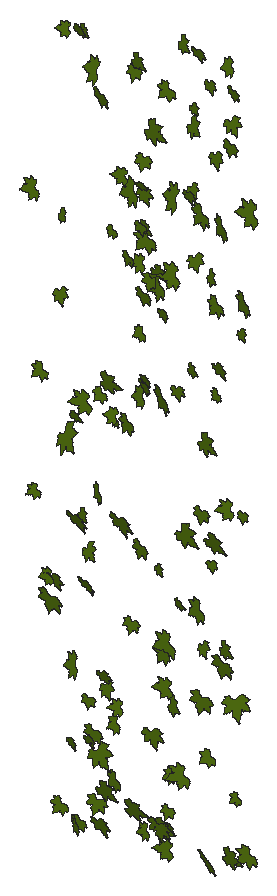
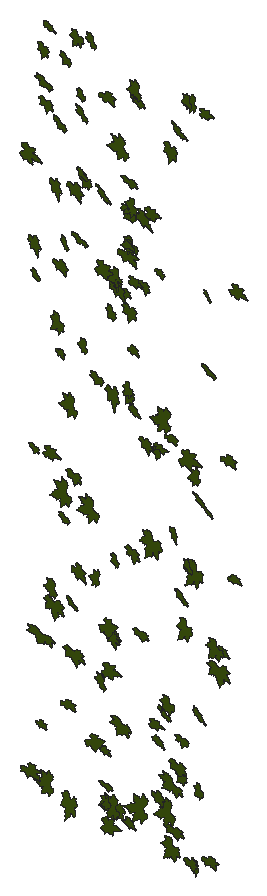
# SketchUp Ruby script. Lengths in inches.
U = 1.inch
M = Sketchup.active_model
def pt(a) = Geom::Point3d.new(a.map { |v| v * U })
def face(e, loops, mat)
  f = e.add_face(loops[0].map { |a| pt(a) })
  loops[1..].each { |l| e.add_face(l.map { |a| pt(a) }).erase! }
  f.material = f.back_material = mat if mat
  f
end
# faces: each face lists its corners as indices into pts; further lists are holes
def faces(e, pts, list, mat = nil) = list.each { |f| face(e, (f[0].is_a?(Array) ? f : [f]).map { |l| l.map { |i| pts[i] } }, mat) }
# xy, xz, yz: faces in a plane at the given z, y or x. An outline is a flat list of corners, or four numbers for a rectangle; further outlines are holes
def ring(l) = l.size == 4 ? [[l[0], l[1]], [l[2], l[1]], [l[2], l[3]], [l[0], l[3]]] : l.each_slice(2).to_a
def flat(e, list, mat, &to3) = list.each { |f| face(e, (f[0].is_a?(Array) ? f : [f]).map { |l| ring(l).map { |u, v| to3.(u, v) } }, mat) }
def xy(e, z, list, mat = nil) = flat(e, list, mat) { |x, y| [x, y, z] }
def xz(e, y, list, mat = nil) = flat(e, list, mat) { |x, z| [x, y, z] }
def yz(e, x, list, mat = nil) = flat(e, list, mat) { |y, z| [x, y, z] }
def lines(e, pts, list) = list.each { |a, b| e.add_line(pt(pts[a]), pt(pts[b])) }
# prism: a flat outline (further loops are holes) pulled along v
def prism(e, loops, v, mat = nil)
  f = face(e, loops, mat); d = Geom::Vector3d.new(v.map { |x| x * U })
  f.pushpull(f.normal.samedirection?(d) ? d.length : -d.length)
end
def box(e, o, s, mat = nil) = prism(e, [[o, [o[0] + s[0], o[1], o[2]], [o[0] + s[0], o[1] + s[1], o[2]], [o[0], o[1] + s[1], o[2]]]], [0, 0, s[2]], mat)
def at(x, y, z, deg = 0) = Geom::Transformation.translation(pt([x, y, z])) * Geom::Transformation.rotation(ORIGIN, Z_AXIS, deg.degrees)
def axes(o, x, y, z) = Geom::Transformation.new([*x, 0, *y, 0, *z, 0, *pt(o).to_a, 1])
def part(name) = M.definitions.add(name)
# library, detail: a bought-in or finely detailed component or shape, given as its bounding box
def library(name, o, s) = part(name).tap { |d| box(d.entities, o, s) }
def detail(e, o, s) = box(e.add_group.entities, o, s)
def put(e, d, t, mat = nil) = e.add_instance(d, t).tap { |i| i.material = mat if mat }
def group(e, t, mat = nil) = e.add_group.tap { |g| g.transformation = t; g.material = mat if mat }.entities
root = M.entities
M.materials.add("[Vegetation Blur 03]").color = [83, 114, 18]
c1 = part("ivy")
xy(c1.entities,0,[[0.782,0,0.786,0,0.787,0.005,0.789,0.009,0.821,0.072,0.875,0.147,1.001,0.272,1.073,0.331,1.137,0.363,1.178,0.379,1.223,0.384,1.272,0.383,1.311,0.374,1.36,0.355,1.399,0.334,1.491,0.285,1.541,0.244,1.583,0.199,1.617,0.15,1.64,0.128,1.662,0.115,1.717,0.105,1.745,0.093,1.784,0.054,1.819,0.057,1.854,0.064,1.882,0.075,1.896,0.074,1.91,0.071,1.937,0.063,1.964,0.053,1.99,0.038,2.016,0.015,2.034,0.002,2.04,0,2.038,0.003,2.036,0.007,2.033,0.038,2.036,0.068,2.045,0.1,2.055,0.116,2.064,0.123,2.077,0.129,2.088,0.129,2.106,0.132,2.118,0.13,2.179,0.132,2.207,0.133,2.225,0.133,2.242,0.138,2.22,0.162,2.207,0.186,2.206,0.213,2.212,0.236,2.228,0.262,2.247,0.274,2.298,0.283,2.355,0.294,2.37,0.296,2.376,0.295,2.377,0.3,2.377,0.303,2.385,0.329,2.411,0.37,2.426,0.392,2.449,0.407,2.511,0.426,2.561,0.444,2.619,0.466,2.589,0.469,2.561,0.476,2.501,0.5,2.449,0.516,2.424,0.523,2.401,0.535,2.377,0.556,2.372,0.568,2.36,0.575,2.268,0.586,2.225,0.592,2.207,0.599,2.194,0.61,2.143,0.65,2.13,0.664,2.122,0.682,2.123,0.7,2.13,0.719,2.148,0.75,2.17,0.781,2.195,0.807,2.221,0.828,2.284,0.874,2.291,0.88,2.288,0.887,2.276,0.9,2.267,0.916,2.265,0.933,2.273,0.967,2.292,1.002,2.313,1.03,2.334,1.054,2.348,1.067,2.358,1.074,2.363,1.076,2.362,1.081,2.35,1.094,2.347,1.11,2.35,1.143,2.359,1.18,2.385,1.254,2.415,1.324,2.448,1.393,2.45,1.4,2.446,1.398,2.44,1.394,2.427,1.383,2.402,1.36,2.376,1.339,2.345,1.324,2.305,1.309,2.282,1.303,2.273,1.306,2.245,1.294,2.212,1.287,2.187,1.291,2.163,1.301,2.142,1.316,2.134,1.327,2.124,1.325,2.09,1.292,2.053,1.259,2.014,1.234,1.973,1.215,1.954,1.21,1.931,1.208,1.909,1.212,1.893,1.22,1.879,1.233,1.872,1.248,1.867,1.281,1.864,1.319,1.821,1.258,1.773,1.197,1.726,1.141,1.698,1.121,1.679,1.116,1.666,1.117,1.647,1.122,1.632,1.129,1.62,1.141,1.617,1.154,1.617,1.219,1.621,1.254,1.623,1.268,1.623,1.281,1.618,1.314,1.606,1.346,1.603,1.375,1.607,1.403,1.603,1.467,1.599,1.499,1.605,1.525,1.614,1.552,1.629,1.577,1.635,1.589,1.629,1.587,1.618,1.582,1.596,1.566,1.581,1.556,1.568,1.552,1.557,1.55,1.545,1.553,1.531,1.562,1.522,1.572,1.504,1.591,1.486,1.611,1.474,1.631,1.457,1.666,1.455,1.684,1.457,1.698,1.452,1.715,1.444,1.728,1.424,1.754,1.419,1.772,1.423,1.786,1.434,1.819,1.444,1.848,1.446,1.855,1.44,1.861,1.43,1.867,1.386,1.904,1.349,1.948,1.326,1.973,1.31,1.995,1.288,2.048,1.284,2.153,1.287,2.254,1.284,2.255,1.282,2.253,1.278,2.247,1.274,2.237,1.266,2.216,1.226,2.125,1.208,2.076,1.184,2.033,1.155,1.984,1.135,1.942,1.111,1.899,1.083,1.861,1.053,1.85,1.059,1.83,1.061,1.809,1.056,1.79,1.049,1.767,1.04,1.749,1.018,1.733,0.994,1.726,0.942,1.734,0.95,1.6875,0.944,1.645,0.932,1.608,0.911,1.585,0.881,1.58,0.854,1.582,0.828,1.588,0.785,1.618,0.773,1.625,0.775,1.614,0.779,1.598,0.796,1.502,0.818,1.402,0.861,1.283,0.882,1.224,0.894,1.174,0.892,1.148,0.886,1.123,0.881,1.107,0.872,1.099,0.849,1.094,0.818,1.092,0.789,1.098,0.762,1.107,0.753,1.113,0.721,1.139,0.698,1.163,0.678,1.194,0.665,1.224,0.628,1.28,0.612,1.312,0.606,1.327,0.606,1.314,0.599,1.282,0.594,1.267,0.581,1.256,0.544,1.245,0.512,1.244,0.473,1.249,0.444,1.256,0.382,1.288,0.339,1.306,0.324,1.316,0.317,1.324,0.309,1.326,0.27,1.314,0.227,1.313,0.185,1.3125,0.152,1.317,0.122,1.328,0.092,1.345,0.073,1.353,0.079,1.338,0.092,1.308,0.117,1.249,0.13,1.215,0.139,1.164,0.147,1.148,0.157,1.136,0.163,1.122,0.174,1.086,0.177,1.067,0.182,1.054,0.186,1.043,0.191,1.038,0.211,1.028,0.237,1.005,0.25,0.974,0.253,0.96,0.25,0.944,0.242,0.914,0.243,0.906,0.249,0.902,0.26,0.894,0.289,0.88,0.307,0.873,0.322,0.862,0.364,0.799,0.403,0.738,0.431,0.709,0.439,0.691,0.441,0.678,0.4375,0.66,0.428,0.645,0.394,0.623,0.303,0.594,0.255,0.581,0.214,0.577,0.179,0.573,0.173,0.568,0.175,0.561,0.167,0.55,0.141,0.523,0.113,0.503,0.077,0.49,0.045,0.486,0.026,0.485,0.019,0.486,0.011,0.483,0,0.471,0.014,0.467,0.044,0.455,0.058,0.447,0.07,0.438,0.097,0.411,0.125,0.394,0.158,0.377,0.174,0.366,0.182,0.359,0.185,0.361,0.242,0.331,0.253,0.316,0.258,0.303,0.262,0.283,0.274,0.278,0.308,0.274,0.341,0.252,0.366,0.226,0.366,0.222,0.37,0.22,0.38,0.221,0.395,0.221,0.425,0.216,0.45,0.207,0.465,0.192,0.473,0.178,0.484,0.15,0.489,0.116,0.483,0.089,0.468,0.058,0.45,0.035,0.435,0.018,0.429,0.011,0.434,0.012,0.438,0.014,0.469,0.019,0.542,0.016,0.581,0.015,0.612,0.027,0.68,0.055,0.696,0.057,0.712,0.052,0.73,0.045,0.741,0.036,0.766,0.014]])
put(root,c1,axes([124.42,173.8,43.62],[0.34903,-0.06561,0.18456],[0.21828,-0.15404,-0.28357],[-0.06714,-0.84183,0.0375]),"[Vegetation Blur 03]")
put(root,c1,axes([125.8,173.8,49.1875],[0.2034,-0.19719,-0.25526],[-0.32297,-0.00076,-0.17132],[-0.05192,-0.76775,0.06573]),"[Vegetation Blur 03]")
put(root,c1,axes([116.46,173.8,6.22],[0.37274,-0.27698,-0.10257],[-0.11734,0.09274,-0.32343],[-0.14192,-0.80413,-0.00197]),"[Vegetation Blur 03]")
put(root,c1,axes([116.69,173.8,14.82],[0.25932,-0.29593,-0.35358],[-0.43934,0.11655,-0.22996],[-0.12392,-1.03246,0.07539]),"[Vegetation Blur 03]")
put(root,c1,axes([124.1,173.8,23.1],[0.31154,-0.18802,0.42817],[0.53015,-0.00865,-0.25753],[-0.0503,-1.25557,-0.06234]),"[Vegetation Blur 03]")
put(root,c1,axes([119.76,173.8,46.72],[0.38042,-0.08348,0.02066],[0.01844,-0.12918,-0.30833],[-0.04412,-0.77385,0.04924]),"[Vegetation Blur 03]")
put(root,c1,axes([118.97,173.8,12.375],[0.28202,-0.18926,-0.22565],[-0.28437,-0.00619,-0.23592],[-0.06351,-0.81269,0.05435]),"[Vegetation Blur 03]")
put(root,c1,axes([122.53,173.8,19.22],[0.06463,-0.12992,0.26421],[0.32679,-0.06667,-0.0584],[-0.04465,-0.67604,-0.04502]),"[Vegetation Blur 03]")
put(root,c1,axes([120.07,173.8,21.99],[0.46442,-0.17928,-0.04706],[-0.05947,-0.00913,-0.38545],[-0.0859,-0.96299,0.01241]),"[Vegetation Blur 03]")
put(root,c1,axes([119.96,173.8,40.93],[0.36429,-0.26691,-0.39719],[-0.49048,0.09297,-0.30946],[-0.1145,-1.24751,0.06192]),"[Vegetation Blur 03]")
put(root,c1,axes([123.74,173.8,40.94],[0.49987,-0.22483,-0.22694],[-0.27931,0.04426,-0.41667],[-0.10606,-1.17624,0.0277]),"[Vegetation Blur 03]")
put(root,c1,axes([115.42,173.8,25.39],[0.26041,0.16269,0.49935],[0.59768,-0.40532,-0.18684],[-0.15294,-1.30696,0.1201]),"[Vegetation Blur 03]")
put(root,c1,axes([118.02,173.8,13.44],[0.29238,-0.00543,0.2431],[0.28843,-0.20948,-0.23179],[-0.07444,-0.83296,0.05671]),"[Vegetation Blur 03]")
put(root,c1,axes([119.89,173.8,46.71],[0.15082,-0.08194,0.36497],[0.44384,-0.11913,-0.12637],[-0.06768,-0.96384,-0.01541]),"[Vegetation Blur 03]")
put(root,c1,axes([124.54,173.8,32.62],[0.36896,-0.184,0.21842],[0.27276,0.00042,-0.30684],[-0.07226,-0.93795,-0.04299]),"[Vegetation Blur 03]")
put(root,c1,axes([121.36,173.8,36.52],[0.43677,-0.25618,-0.34823],[-0.42807,0.08886,-0.36791],[-0.11962,-1.25334,0.04509]),"[Vegetation Blur 03]")
put(root,c1,axes([122.84,173.8,11.16],[0.31711,-0.08877,-0.37028],[-0.45541,-0.10498,-0.25583],[0.01733,-1.13422,0.05266]),"[Vegetation Blur 03]")
put(root,c1,axes([123.75,173.8,27.99],[0.19561,-0.07372,0.44835],[0.54629,-0.12238,-0.16192],[-0.06809,-1.19373,-0.01109]),"[Vegetation Blur 03]")
put(root,c1,axes([119.37,173.8,28.36],[0.44792,-0.20906,-0.13241],[-0.16237,0.03502,-0.37455],[-0.10139,-0.9797,0.01487]),"[Vegetation Blur 03]")
put(root,c1,axes([121.4,173.8,34.4],[0.29752,-0.1463,0.14185],[0.17418,-0.03541,-0.24908],[-0.07018,-0.70816,-0.01685]),"[Vegetation Blur 03]")
put(root,c1,axes([120.28,173.8,30.4],[0.3929,-0.21833,0.06927],[0.09371,0.04854,-0.33],[-0.09838,-0.82573,-0.03771]),"[Vegetation Blur 03]")
put(root,c1,axes([121.45,173.8,17.06],[0.4568,-0.18649,-0.14633],[-0.18134,0.01163,-0.3794],[-0.08646,-1.00976,0.02265]),"[Vegetation Blur 03]")
put(root,c1,axes([124.15,173.8,47.36],[0.32177,-0.10077,0.13804],[0.16444,-0.08743,-0.26534],[-0.06299,-0.74292,0.0125]),"[Vegetation Blur 03]")
put(root,c1,axes([125.04,173.8,17.66],[0.12722,-0.05638,0.35512],[0.42991,-0.13892,-0.10606],[-0.07252,-0.92248,-0.00573]),"[Vegetation Blur 03]")
put(root,c1,axes([120.51,173.8,38.51],[0.49046,-0.12487,-0.25125],[-0.31171,-0.05916,-0.40067],[-0.03597,-1.19015,0.04628]),"[Vegetation Blur 03]")
put(root,c1,axes([117.45,173.8,7.7],[0.48615,-0.06506,-0.03255],[-0.04363,-0.12709,-0.39413],[-0.0262,-0.99568,0.05243]),"[Vegetation Blur 03]")
put(root,c1,axes([122.54,173.8,37.27],[0.22309,-0.1604,-0.43567],[-0.53899,-0.01598,-0.18291],[-0.02282,-1.19045,0.06116]),"[Vegetation Blur 03]")
put(root,c1,axes([115.29,173.8,33.23],[0.32579,-0.0019,0.20222],[0.24053,-0.19974,-0.25841],[-0.05947,-0.81825,0.06261]),"[Vegetation Blur 03]")
put(root,c1,axes([121.23,173.8,20.77],[0.18692,-0.08145,0.20202],[0.24238,-0.1034,-0.15594],[-0.06396,-0.62987,-0.00053]),"[Vegetation Blur 03]")
put(root,c1,axes([124.66,173.8,36.38],[0.42696,-0.16855,-0.18226],[-0.22665,-0.00186,-0.3534],[-0.07216,-0.99152,0.03164]),"[Vegetation Blur 03]")
put(root,c1,axes([120.22,173.8,42.21],[0.40348,-0.0468,0.02113],[0.02171,-0.14086,-0.32526],[-0.02676,-0.81998,0.05467]),"[Vegetation Blur 03]")
put(root,c1,axes([125.29,173.8,6.73],[0.10484,-0.11239,0.45286],[0.55605,-0.06423,-0.08825],[-0.04094,-1.16025,-0.03898]),"[Vegetation Blur 03]")
put(root,c1,axes([120.62,173.8,37.02],[0.14335,-0.13764,-0.29117],[-0.36286,-0.03379,-0.11648],[-0.00945,-0.79049,0.05568]),"[Vegetation Blur 03]")
put(root,c1,axes([116.05,173.8,10.03],[0.27088,-0.15261,0.15464],[0.19269,-0.01614,-0.22733],[-0.06536,-0.68006,-0.0293]),"[Vegetation Blur 03]")
put(root,c1,axes([123.76,173.8,17.52],[0.23663,-0.00308,0.21961],[0.25991,-0.18831,-0.18695],[-0.06967,-0.71292,0.04843]),"[Vegetation Blur 03]")
put(root,c1,axes([121.78,173.8,8.61],[0.33968,-0.06301,-0.00772],[-0.01455,-0.11855,-0.2742],[-0.02856,-0.68915,0.04788]),"[Vegetation Blur 03]")
put(root,c1,axes([125.75,173.8,25.94],[0.1638,-0.10041,-0.33523],[-0.41333,-0.07495,-0.13099],[0.01603,-0.90688,0.04794]),"[Vegetation Blur 03]")
put(root,c1,axes([119.59,173.8,7.26],[0.11966,-0.19885,0.48664],[0.60405,0.04067,-0.09632],[0.00062,-1.25082,-0.0805]),"[Vegetation Blur 03]")
put(root,c1,axes([123.46,173.8,15.29],[0.58789,-0.11281,-0.04556],[-0.05859,-0.05769,-0.48112],[-0.05185,-1.21383,0.0271]),"[Vegetation Blur 03]")
put(root,c1,axes([124.32,173.8,36.93],[0.07908,0.01608,0.29029],[0.3424,-0.20709,-0.06032],[-0.09663,-0.72064,0.02381]),"[Vegetation Blur 03]")
put(root,c1,axes([116.74,173.8,21.9],[0.13772,-0.02232,0.26418],[0.31478,-0.16115,-0.11144],[-0.07624,-0.70573,0.01709]),"[Vegetation Blur 03]")
put(root,c1,axes([119.34,173.8,13.22],[0.11929,-0.10597,-0.2818],[-0.34889,-0.06251,-0.09467],[0.01224,-0.74914,0.04776]),"[Vegetation Blur 03]")
put(root,c1,axes([119.16,173.8,28.375],[0.04403,-0.12753,-0.27738],[-0.34532,-0.03734,-0.03381],[0.01033,-0.70424,0.05202]),"[Vegetation Blur 03]")
put(root,c1,axes([124.35,173.8,12.46],[0.296,-0.08214,-0.20649],[-0.25613,-0.08908,-0.23898],[-0.00188,-0.79632,0.04803]),"[Vegetation Blur 03]")
put(root,c1,axes([116.8,173.8,47.37],[0.14289,-0.07488,0.25812],[0.31299,-0.09737,-0.11985],[-0.0582,-0.70749,-0.01082]),"[Vegetation Blur 03]")
put(root,c1,axes([122.61,173.8,48.58],[0.1212,0.00874,0.32904],[0.39357,-0.19062,-0.09576],[-0.08752,-0.84508,0.025]),"[Vegetation Blur 03]")
put(root,c1,axes([117.67,173.8,44.84],[0.50217,-0.23211,-0.02067],[-0.01614,0.08923,-0.41886],[-0.11447,-1.03084,-0.03161]),"[Vegetation Blur 03]")
put(root,c1,axes([119.54,173.8,17.7],[0.40879,-0.06868,-0.00639],[-0.01176,-0.09983,-0.33231],[-0.0322,-0.83542,0.04024]),"[Vegetation Blur 03]")
put(root,c1,axes([115.99,173.8,21.96],[0.55336,-0.2755,0.17895],[0.23761,0.14136,-0.45516],[-0.0977,-1.21665,-0.0934]),"[Vegetation Blur 03]")
put(root,c1,axes([120.64,173.8,36.12],[0.43256,-0.06671,-0.01604],[-0.02325,-0.10108,-0.35159],[-0.02994,-0.88528,0.04135]),"[Vegetation Blur 03]")
put(root,c1,axes([117.74,173.8,7.85],[0.29611,-0.16504,0.41768],[0.51687,0.01316,-0.24325],[-0.03458,-1.21665,-0.05929]),"[Vegetation Blur 03]")
put(root,c1,axes([122.2,173.8,10.68],[0.22279,-0.12525,-0.19809],[-0.24846,-0.03124,-0.18302],[-0.02974,-0.67725,0.04508]),"[Vegetation Blur 03]")
put(root,c1,axes([123.22,173.8,31.7],[0.0683,-0.05119,0.27634],[0.33407,-0.11649,-0.05839],[-0.06049,-0.70118,-0.01047]),"[Vegetation Blur 03]")
put(root,c1,axes([116.51,173.8,47.37],[0.16816,-0.15089,0.24654],[0.3088,-0.00002,-0.1403],[-0.03567,-0.71145,-0.05229]),"[Vegetation Blur 03]")
put(root,c1,axes([116.29,173.8,47.72],[0.09099,-0.0894,-0.27257],[-0.33609,-0.07013,-0.07111],[0.02177,-0.70885,0.04141]),"[Vegetation Blur 03]")
put(root,c1,axes([122.04,173.8,13.59],[0.06873,0.01711,0.34805],[0.41669,-0.19262,-0.05332],[-0.09114,-0.86777,0.0187]),"[Vegetation Blur 03]")
put(root,c1,axes([117.23,173.8,11.3],[0.4987,-0.12613,-0.04723],[-0.0598,-0.02572,-0.40975],[-0.05942,-1.03278,0.01597]),"[Vegetation Blur 03]")
put(root,c1,axes([118.09,173.8,46.43],[0.1383,-0.27518,-0.42018],[-0.52123,0.14835,-0.12955],[-0.10615,-1.08693,0.0887]),"[Vegetation Blur 03]")
put(root,c1,axes([120.29,173.8,38.23],[0.16779,-0.0883,0.30239],[0.37001,-0.06611,-0.13979],[-0.04708,-0.83437,-0.02093]),"[Vegetation Blur 03]")
put(root,c1,axes([121.85,173.8,46.65],[0.37323,-0.08724,-0.21133],[-0.2619,-0.06711,-0.30372],[-0.01607,-0.93236,0.04164]),"[Vegetation Blur 03]")
put(root,c1,axes([123.59,173.8,24.92],[0.43658,-0.10423,0.00392],[0.00224,-0.04583,-0.35826],[-0.05083,-0.89729,0.01784]),"[Vegetation Blur 03]")
put(root,c1,axes([114.26,173.8,22.84],[0.22258,-0.06561,-0.19839],[-0.24493,-0.08915,-0.17839],[0.01076,-0.67235,0.04301]),"[Vegetation Blur 03]")
put(root,c1,axes([117.42,173.8,6.36],[0.49317,-0.18476,0.20262],[0.2548,0.0498,-0.40595],[-0.06909,-1.1351,-0.05079]),"[Vegetation Blur 03]")
put(root,c1,axes([120.14,173.8,40.21],[0.36838,-0.06003,0.20905],[0.25298,-0.09287,-0.30112],[-0.04965,-0.91861,0.01678]),"[Vegetation Blur 03]")
put(root,c1,axes([115.51,173.8,6.9],[0.37574,-0.07096,-0.15978],[-0.19839,-0.07956,-0.3052],[-0.01253,-0.86822,0.04103]),"[Vegetation Blur 03]")
put(root,c1,axes([125.33,173.8,44.77],[0.4277,-0.13208,-0.01923],[-0.02433,-0.00684,-0.35292],[-0.0639,-0.88143,0.00562]),"[Vegetation Blur 03]")
put(root,c1,axes([118.51,173.8,22.8],[0.63866,-0.23189,0.12864],[0.16822,0.10928,-0.52532],[-0.09614,-1.34925,-0.06466]),"[Vegetation Blur 03]")
put(root,c1,axes([120.07,173.8,38.55],[0.32611,-0.0735,0.11387],[0.13621,-0.07341,-0.2673],[-0.04678,-0.72621,0.01549]),"[Vegetation Blur 03]")
put(root,c1,axes([114.25,173.8,38.86],[0.22705,-0.11945,-0.35491],[-0.43835,-0.02,-0.18572],[-0.01818,-1.0093,0.04569]),"[Vegetation Blur 03]")
put(root,c1,axes([123.15,173.8,37.73],[0.33502,0.02499,0.20079],[0.2423,-0.1873,-0.26561],[-0.04435,-0.83458,0.06562]),"[Vegetation Blur 03]")
put(root,c1,axes([124.97,173.8,40.71],[0.46455,-0.28541,-0.24702],[-0.29064,0.17394,-0.39567],[-0.16241,-1.12761,0.00149]),"[Vegetation Blur 03]")
put(root,c1,axes([124.27,173.8,22.22],[0.28684,-0.06236,0.1063],[0.12625,-0.08285,-0.23456],[-0.04409,-0.64295,0.01992]),"[Vegetation Blur 03]")
put(root,c1,axes([117.94,173.8,29.18],[0.29981,-0.06525,-0.13535],[-0.1686,-0.07812,-0.24283],[-0.00912,-0.70071,0.03968]),"[Vegetation Blur 03]")
put(root,c1,axes([122.89,173.8,41.17],[0.34101,-0.13421,0.11002],[0.1371,0.00224,-0.28262],[-0.06025,-0.75456,-0.02041]),"[Vegetation Blur 03]")
put(root,c1,axes([126.56,173.8,8.21],[0.3982,-0.07833,-0.27853],[-0.34327,-0.06231,-0.32413],[-0.0091,-1.07738,0.039]),"[Vegetation Blur 03]")
put(root,c1,axes([126.05,173.8,34.78],[0.19571,-0.04059,0.18321],[0.21938,-0.10557,-0.15978],[-0.05153,-0.6037,0.01562]),"[Vegetation Blur 03]")
put(root,c1,axes([126.14,173.8,25.49],[0.2893,-0.06946,0.05279],[0.06075,-0.07196,-0.23668],[-0.04039,-0.60575,0.02206]),"[Vegetation Blur 03]")
put(root,c1,axes([116.96,173.8,20.09],[0.20883,0.04815,0.31421],[0.37772,-0.20796,-0.1622],[-0.0781,-0.87697,0.05572]),"[Vegetation Blur 03]")
put(root,c1,axes([116.29,173.8,26.97],[0.1451,-0.1312,0.25798],[0.3214,0.00081,-0.12034],[-0.02623,-0.71573,-0.04743]),"[Vegetation Blur 03]")
put(root,c1,axes([122.73,173.8,41.38],[0.14321,-0.30149,-0.44399],[-0.54717,0.20081,-0.13901],[-0.13425,-1.14006,0.09293]),"[Vegetation Blur 03]")
put(root,c1,axes([114.48,173.8,29.33],[0.3254,-0.08509,-0.21734],[-0.269,-0.05049,-0.26515],[-0.01633,-0.86378,0.03691]),"[Vegetation Blur 03]")
put(root,c1,axes([120.98,173.8,36.26],[0.26264,-0.10696,0.28896],[0.35555,-0.0243,-0.21667],[-0.0405,-0.90682,-0.02828]),"[Vegetation Blur 03]")
put(root,c1,axes([118.64,173.8,37.94],[0.27643,-0.11245,-0.0959],[-0.1208,-0.01738,-0.22873],[-0.04691,-0.61786,0.02389]),"[Vegetation Blur 03]")
put(root,c1,axes([121.35,173.8,30.54],[0.55558,-0.31709,-0.23093],[-0.26347,0.22092,-0.46992],[-0.18545,-1.26384,-0.0242]),"[Vegetation Blur 03]")
put(root,c1,axes([116.6875,173.8,18.76],[0.46892,-0.24319,0.11777],[0.16224,0.13537,-0.38629],[-0.09203,-1.00049,-0.08089]),"[Vegetation Blur 03]")
put(root,c1,axes([126.25,173.8,37.14],[0.45147,-0.25025,-0.22719],[-0.26949,0.14362,-0.38159],[-0.1402,-1.08195,0.00189]),"[Vegetation Blur 03]")
put(root,c1,axes([120.36,173.8,30.58],[0.28308,-0.16005,0.12566],[0.16212,0.03888,-0.23548],[-0.05892,-0.66197,-0.04421]),"[Vegetation Blur 03]")
put(root,c1,axes([124.67,173.8,17.57],[0.60359,-0.16861,-0.0634],[-0.07511,0.04962,-0.497],[-0.08431,-1.25133,-0.01117]),"[Vegetation Blur 03]")
put(root,c1,axes([117.05,173.8,10.5],[0.29444,-0.13699,0.14225],[0.1786,0.0132,-0.24425],[-0.05394,-0.70397,-0.03226]),"[Vegetation Blur 03]")
put(root,c1,axes([121.74,173.8,7.37],[0.20518,-0.11933,0.20995],[0.26085,-0.0065,-0.17038],[-0.03866,-0.67709,-0.03537]),"[Vegetation Blur 03]")
put(root,c1,axes([123.75,173.8,20.17],[0.36665,-0.19895,-0.32997],[-0.4044,0.08632,-0.30749],[-0.09631,-1.11984,0.03492]),"[Vegetation Blur 03]")
put(root,c1,axes([125.54,173.8,47.62],[0.38177,-0.16884,0.00908],[0.01686,0.05275,-0.31784],[-0.08106,-0.78418,-0.02334]),"[Vegetation Blur 03]")
put(root,c1,axes([123.1,173.8,44.37],[0.13518,0.07282,0.36034],[0.43243,-0.22734,-0.10083],[-0.09589,-0.9226,0.05329]),"[Vegetation Blur 03]")
put(root,c1,axes([116.58,173.8,6.29],[0.37414,-0.10141,-0.07585],[-0.09511,-0.0243,-0.3074],[-0.04493,-0.79294,0.01912]),"[Vegetation Blur 03]")
put(root,c1,axes([119.47,173.8,36.87],[0.35103,-0.1488,-0.07514],[-0.0909,0.03087,-0.29249],[-0.07377,-0.74614,0.00288]),"[Vegetation Blur 03]")
put(root,c1,axes([120.84,173.8,7.66],[0.62439,-0.15847,0.04406],[0.05688,0.04229,-0.51297],[-0.0749,-1.28898,-0.02225]),"[Vegetation Blur 03]")
put(root,c1,axes([122.37,173.8,22.82],[0.30964,-0.0676,0.45983],[0.56279,-0.06237,-0.25387],[-0.0424,-1.3215,-0.01154]),"[Vegetation Blur 03]")
put(root,c1,axes([115.61,173.8,37.17],[0.07732,0.04701,0.24249],[0.28519,-0.19481,-0.05463],[-0.0864,-0.60099,0.03668]),"[Vegetation Blur 03]")
put(root,c1,axes([123.26,173.8,45.61],[0.18338,-0.0476,0.19783],[0.23906,-0.08339,-0.15076],[-0.04624,-0.61987,0.00509]),"[Vegetation Blur 03]")
put(root,c1,axes([118.13,173.8,29.11],[0.08822,-0.12322,0.46198],[0.56917,0.00464,-0.0722],[-0.00698,-1.17889,-0.04857]),"[Vegetation Blur 03]")
put(root,c1,axes([122.2,173.8,15.32],[0.10909,-0.05884,-0.38294],[-0.46937,-0.06819,-0.08742],[0.02587,-0.98895,0.02881]),"[Vegetation Blur 03]")
put(root,c1,axes([118.81,173.8,9.4],[0.34978,-0.17504,-0.23097],[-0.28247,0.06704,-0.29293],[-0.08681,-0.92345,0.02252]),"[Vegetation Blur 03]")
put(root,c1,axes([127.17,173.8,42.125],[0.18243,-0.13935,-0.48722],[-0.59996,0.02639,-0.15082],[-0.03212,-1.28429,0.04976]),"[Vegetation Blur 03]")
put(root,c1,axes([121.99,173.8,17.83],[0.34831,-0.13161,-0.42418],[-0.52189,0.01831,-0.28634],[-0.04303,-1.28736,0.03929]),"[Vegetation Blur 03]")
put(root,c1,axes([117.88,173.8,24.12],[0.31941,-0.24553,-0.21108],[-0.24847,0.1507,-0.27802],[-0.13923,-0.8322,0.01193]),"[Vegetation Blur 03]")
put(root,c1,axes([126.01,173.8,10.74],[0.21979,-0.07452,-0.15702],[-0.1954,-0.04663,-0.1787],[-0.01213,-0.59927,0.03343]),"[Vegetation Blur 03]")
put(root,c1,axes([120.59,173.8,30.09],[0.18991,-0.19032,-0.31472],[-0.38839,0.08836,-0.16451],[-0.08006,-0.88012,0.05154]),"[Vegetation Blur 03]")
put(root,c1,axes([120.78,173.8,7.31],[0.2031,-0.14404,-0.26055],[-0.32267,0.0347,-0.17055],[-0.052,-0.77785,0.04064]),"[Vegetation Blur 03]")
put(root,c1,axes([123.11,173.8,41.29],[0.21707,0.00977,0.22202],[0.26718,-0.14285,-0.17301],[-0.05136,-0.70178,0.03831]),"[Vegetation Blur 03]")
put(root,c1,axes([120.61,173.8,43.19],[0.18628,-0.03587,0.49266],[0.60208,-0.08964,-0.15266],[-0.04677,-1.29689,-0.00307]),"[Vegetation Blur 03]")
put(root,c1,axes([120.45,173.8,33.25],[0.22039,-0.10268,-0.20891],[-0.2592,-0.01,-0.18136],[-0.02883,-0.69502,0.03347]),"[Vegetation Blur 03]")
put(root,c1,axes([115.13,173.8,18.67],[0.1748,-0.10036,-0.26156],[-0.32362,-0.01023,-0.14344],[-0.01895,-0.75115,0.0369]),"[Vegetation Blur 03]")
put(root,c1,axes([114.51,173.8,17.55],[0.65346,-0.15996,-0.07236],[-0.08578,0.05992,-0.53686],[-0.0809,-1.3557,-0.01519]),"[Vegetation Blur 03]")
put(root,c1,axes([118.73,173.8,27.98],[0.28723,-0.15203,-0.02555],[-0.02588,0.0511,-0.24162],[-0.07595,-0.59236,-0.01429]),"[Vegetation Blur 03]")
put(root,c1,axes([125.13,173.8,15.34],[0.58242,0.07305,0.2372],[0.29248,-0.20649,-0.46835],[-0.01349,-1.32342,0.08617]),"[Vegetation Blur 03]")
put(root,c1,axes([117.21,173.8,9.65],[0.43574,0.04341,0.40329],[0.4922,-0.17124,-0.35133],[-0.04861,-1.34487,0.05775]),"[Vegetation Blur 03]")
put(root,c1,axes([117.33,173.8,28.72],[0.17219,-0.03701,-0.43547],[-0.53302,-0.07752,-0.13935],[0.03036,-1.15115,0.02338]),"[Vegetation Blur 03]")
put(root,c1,axes([125.23,173.8,45.55],[0.34233,0.0367,0.25351],[0.30852,-0.16299,-0.27378],[-0.04025,-0.93715,0.05755]),"[Vegetation Blur 03]")
put(root,c1,axes([120.4375,173.8,12.09],[0.51003,-0.05161,0.17077],[0.20792,-0.06034,-0.4165],[-0.03431,-1.13281,0.01441]),"[Vegetation Blur 03]")
put(root,c1,axes([122.27,173.8,6.81],[0.07011,-0.04175,-0.39035],[-0.47768,-0.07166,-0.05594],[0.03155,-0.99215,0.02047]),"[Vegetation Blur 03]")
put(root,c1,axes([123.36,173.8,48.86],[0.38814,-0.14356,0.10109],[0.12917,0.04667,-0.31993],[-0.05936,-0.83711,-0.03517]),"[Vegetation Blur 03]")
put(root,c1,axes([120.17,173.8,35.22],[0.46399,-0.15608,-0.0301],[-0.03246,0.06122,-0.3832],[-0.07784,-0.95586,-0.01963]),"[Vegetation Blur 03]")
put(root,c1,axes([124.79,173.8,31.49],[0.2496,-0.10992,-0.13236],[-0.16418,0.00788,-0.20725],[-0.04691,-0.61248,0.02109]),"[Vegetation Blur 03]")
put(root,c1,axes([121.25,173.8,6.9],[0.12855,-0.09811,0.43066],[0.52964,-0.00555,-0.1055],[-0.01392,-1.1176,-0.03728]),"[Vegetation Blur 03]")
put(root,c1,axes([123.75,173.8,7.04],[0.61856,-0.3329,-0.06965],[-0.05285,0.26763,-0.51381],[-0.1751,-1.25675,-0.09097]),"[Vegetation Blur 03]")
put(root,c1,axes([122.17,173.8,30.63],[0.33984,-0.05336,0.11192],[0.13528,-0.05673,-0.27786],[-0.03432,-0.75199,0.01302]),"[Vegetation Blur 03]")
put(root,c1,axes([117.78,173.8,14.15],[0.36419,-0.14328,0.1768],[0.2225,0.04791,-0.29916],[-0.04769,-0.87068,-0.04556]),"[Vegetation Blur 03]")
put(root,c1,axes([119.65,173.8,41.16],[0.05825,-0.05857,-0.32384],[-0.39732,-0.0501,-0.04618],[0.02002,-0.82377,0.02584]),"[Vegetation Blur 03]")
put(root,c1,axes([120.08,173.8,40.54],[0.28631,-0.17737,0.19402],[0.25002,0.08801,-0.2331],[-0.03783,-0.76071,-0.07221]),"[Vegetation Blur 03]")
put(root,c1,axes([117.02,173.8,12.71],[0.35341,-0.05372,0.02619],[0.03014,-0.05475,-0.28854],[-0.02834,-0.72817,0.01976]),"[Vegetation Blur 03]")
put(root,c1,axes([114.76,173.8,18.26],[0.44883,-0.14962,0.17944],[0.22549,0.05754,-0.36812],[-0.05276,-1.02686,-0.04677]),"[Vegetation Blur 03]")
